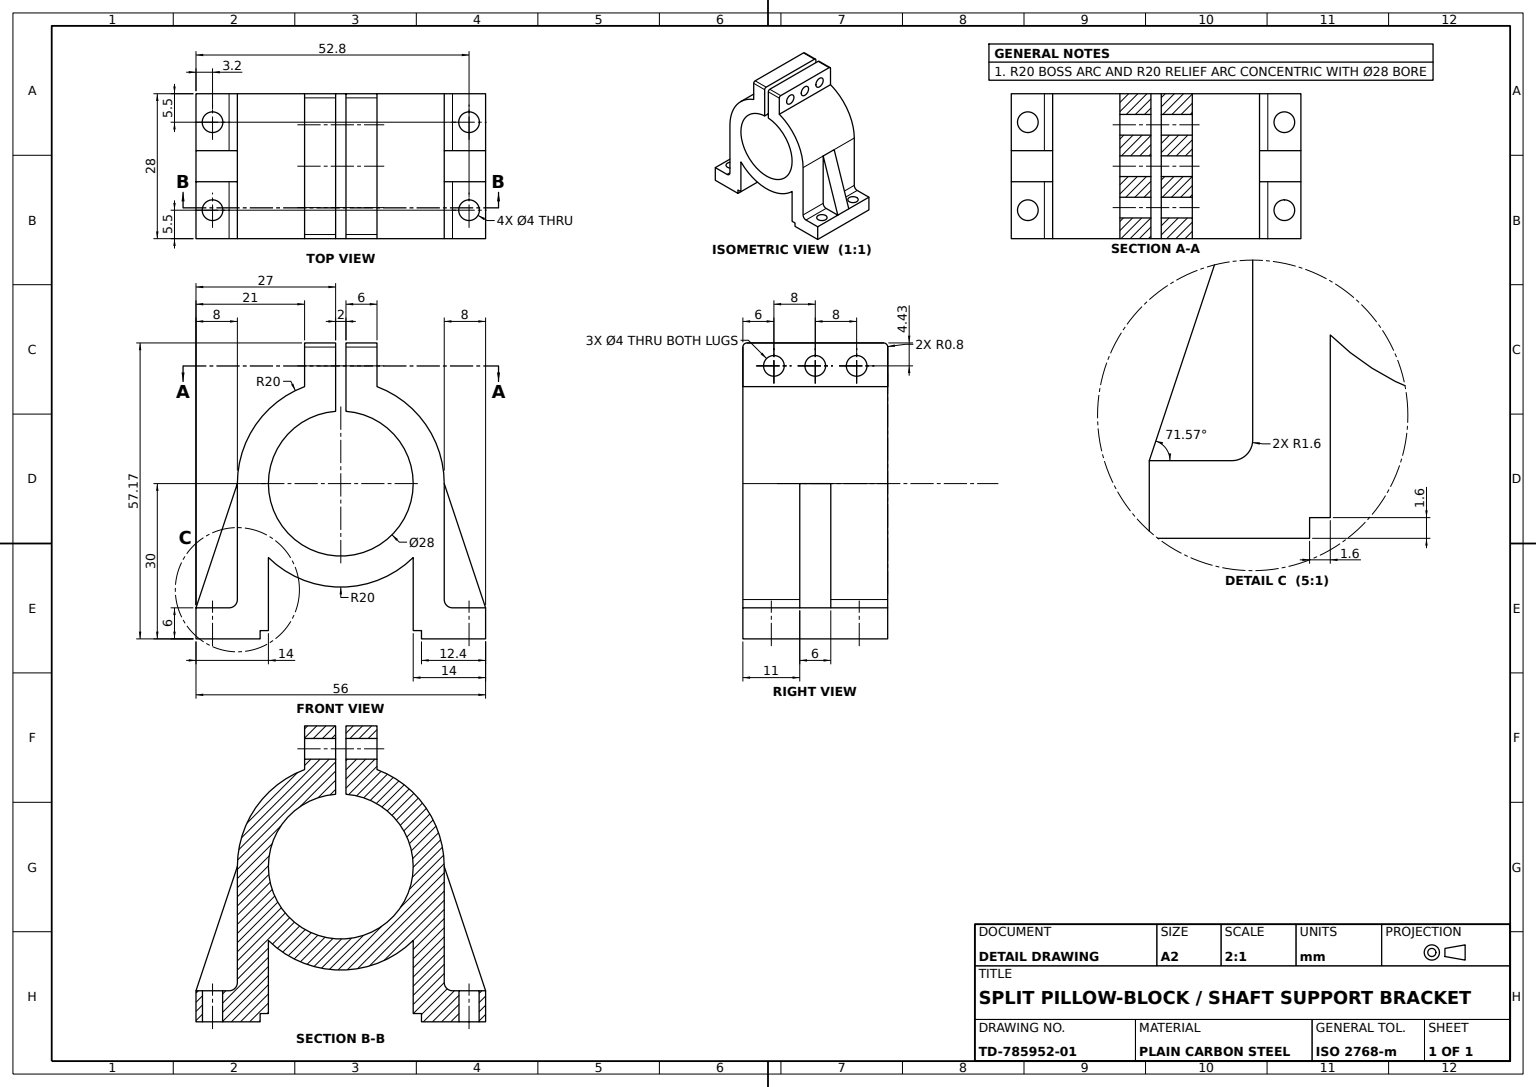
solid
v1 (-20,0,28)
v2 (-20,0,17)
e1 v1 v2 LINE
v3 (-20,-22.4,17)
e2 v3 v2 LINE
v4 (-20,-22.4,28)
e3 v3 v4 LINE
e4 v4 v1 LINE
face PLANE(AX(P(-20,0,17),D(1,0,0),D(0,0,-1))) rev [e1 -e2 e3 e4]
v5 (-28,-24,28)
v6 (-28,-24,17)
e5 v5 v6 LINE
v7 (-28,-24,11)
e6 v6 v7 LINE
v8 (-28,-24,0)
e7 v7 v8 LINE
v9 (-28,-30,0)
e8 v8 v9 LINE
v10 (-28,-30,28)
e9 v10 v9 LINE
e10 v5 v10 LINE
face PLANE(AX(P(-28,-24,28),D(1,0,0),D(0,0,-1))) rev [e5 e6 e7 e8 -e9 -e10]
v11 (-21.6,-24,11)
v12 (-21.6,-24,0)
e11 v11 v12 LINE
v13 (-20,-22.4,11)
e12 v13 v11 CIRCLE(AX(P(-21.6,-22.4,11),D(0,0,-1),D(-1,0,0)),1.6)
v14 (-20,-22.4,0)
e13 v13 v14 LINE
e14 v14 v12 CIRCLE(AX(P(-21.6,-22.4,0),D(0,0,-1),D(-1,0,0)),1.6)
face CYL(AX(P(-21.6,-22.4,11),D(0,0,-1),D(-1,0,0)),1.6) rev [-e11 -e12 e13 e14]
v15 (20,-22.4,11)
v16 (20,0,11)
e15 v15 v16 LINE
v17 (20,-22.4,0)
e16 v15 v17 LINE
v18 (20,0,0)
e17 v17 v18 LINE
e18 v16 v18 LINE
face PLANE(AX(P(20,0,11),D(-1,0,0),D(0,0,1))) rev [-e15 e16 e17 -e18]
v19 (1,27.174984,0.8)
v20 (7,27.174984,0.8)
e19 v19 v20 LINE
v21 (7,26.374984,0)
e20 v20 v21 CIRCLE(AX(P(7,26.374984,0.8),D(-1,0,0),D(0,0,-1)),0.8)
v22 (1,26.374984,0)
e21 v21 v22 LINE
e22 v19 v22 CIRCLE(AX(P(1,26.374984,0.8),D(-1,0,0),D(0,0,-1)),0.8)
face CYL(AX(P(-11,26.374984,0.8),D(1,0,0),D(0,0,-1)),0.8) [e19 e20 e21 -e22]
v23 (1,22.743733,4)
v24 (1,22.743733,8)
e23 v23 v24 CIRCLE(AX(P(1,22.743733,6),D(1,0,0),D(0,0,-1)),2)
v25 (7,22.743733,4)
e24 v23 v25 LINE
v26 (7,22.743733,8)
e25 v25 v26 CIRCLE(AX(P(7,22.743733,6),D(1,0,0),D(0,0,-1)),2)
e26 v24 v26 LINE
face CYL(AX(P(-13,22.743733,6),D(1,0,0),D(0,0,-1)),2) rev [-e23 e24 e25 -e26]
v27 (20,-22.4,17)
v28 (20,-22.4,28)
e27 v27 v28 LINE
v29 (21.6,-24,28)
e28 v28 v29 CIRCLE(AX(P(21.6,-22.4,28),D(0,0,1),D(-1,0,0)),1.6)
v30 (21.6,-24,17)
e29 v30 v29 LINE
e30 v27 v30 CIRCLE(AX(P(21.6,-22.4,17),D(0,0,1),D(-1,0,0)),1.6)
face CYL(AX(P(21.6,-22.4,17),D(0,0,1),D(1,0,0)),1.6) rev [e27 e28 -e29 -e30]
v31 (21.6,-24,11)
e31 v31 v15 CIRCLE(AX(P(21.6,-22.4,11),D(0,0,-1),D(-1,0,0)),1.6)
v32 (21.6,-24,0)
e32 v31 v32 LINE
e33 v32 v17 CIRCLE(AX(P(21.6,-22.4,0),D(0,0,-1),D(-1,0,0)),1.6)
face CYL(AX(P(21.6,-22.4,11),D(0,0,-1),D(-1,0,0)),1.6) rev [-e16 -e31 e32 e33]
v33 (24.8,-30,24.5)
v34 (24.8,-24,24.5)
e34 v33 v34 LINE
v35 (24.8,-24,20.5)
e35 v34 v35 CIRCLE(AX(P(24.8,-24,22.5),D(0,1,0),D(0,0,1)),2)
v36 (24.8,-30,20.5)
e36 v36 v35 LINE
e37 v33 v36 CIRCLE(AX(P(24.8,-30,22.5),D(0,1,0),D(0,0,1)),2)
face CYL(AX(P(24.8,-44,22.5),D(0,1,0),D(0,0,1)),2) rev [e34 e35 -e36 -e37]
v37 (28,-24,11)
e38 v16 v37 LINE
v38 (20,0,17)
e39 v38 v16 LINE
v39 (28,-24,17)
e40 v39 v38 LINE
e41 v39 v37 LINE
face PLANE(AX(P(20,0,0),D(0.948683298,0.316227766,0),D(-0.316227766,0.948683298,0))) [-e38 -e39 -e40 e41]
v40 (24.8,-30,3.5)
v41 (24.8,-30,7.5)
e42 v40 v41 CIRCLE(AX(P(24.8,-30,5.5),D(0,1,0),D(0,0,1)),2)
v42 (24.8,-24,3.5)
e43 v40 v42 LINE
v43 (24.8,-24,7.5)
e44 v42 v43 CIRCLE(AX(P(24.8,-24,5.5),D(0,1,0),D(0,0,1)),2)
e45 v41 v43 LINE
face CYL(AX(P(24.8,-44,5.5),D(0,1,0),D(0,0,1)),2) rev [-e42 e43 e44 -e45]
v44 (-14,-14.282857,0)
v45 (14,-14.282857,0)
e46 v44 v45 CIRCLE(AX(P(0,0,0),D(0,0,1),D(1,0,0)),20)
v46 (14,-14.282857,28)
e47 v46 v45 LINE
v47 (-14,-14.282857,28)
e48 v47 v46 CIRCLE(AX(P(0,0,28),D(0,0,1),D(1,0,0)),20)
e49 v47 v44 LINE
face CYL(AX(P(0,0,28),D(0,0,-1),D(-1,0,0)),20) [e46 -e47 -e48 e49]
v48 (-21.6,-24,17)
v49 (-21.6,-24,28)
e50 v48 v49 LINE
e51 v49 v4 CIRCLE(AX(P(-21.6,-22.4,28),D(0,0,1),D(-1,0,0)),1.6)
e52 v48 v3 CIRCLE(AX(P(-21.6,-22.4,17),D(0,0,1),D(-1,0,0)),1.6)
face CYL(AX(P(-21.6,-22.4,17),D(0,0,1),D(1,0,0)),1.6) rev [e50 e51 -e3 -e52]
v50 (-7,26.374984,28)
v51 (-7,27.174984,27.2)
e53 v50 v51 CIRCLE(AX(P(-7,26.374984,27.2),D(-1,0,0),D(0,0,-1)),0.8)
v52 (-1,26.374984,28)
e54 v52 v50 LINE
v53 (-1,27.174984,27.2)
e55 v53 v52 CIRCLE(AX(P(-1,26.374984,27.2),D(1,0,0),D(0,0,1)),0.8)
e56 v51 v53 LINE
face CYL(AX(P(-11,26.374984,27.2),D(1,0,0),D(0,0,-1)),0.8) [-e53 -e54 -e55 -e56]
e57 v35 v34 CIRCLE(AX(P(24.8,-24,22.5),D(0,1,0),D(0,0,1)),2)
v54 (28,-24,28)
e58 v29 v54 LINE
e59 v54 v39 LINE
e60 v30 v39 LINE
face PLANE(AX(P(28,-24,17),D(0,-1,0),D(0,0,-1))) rev [-e35 -e57] [e58 e59 -e60 e29]
e61 v43 v42 CIRCLE(AX(P(24.8,-24,5.5),D(0,1,0),D(0,0,1)),2)
e62 v41 v40 CIRCLE(AX(P(24.8,-30,5.5),D(0,1,0),D(0,0,1)),2)
face CYL(AX(P(24.8,-44,5.5),D(0,1,0),D(0,0,1)),2) rev [e45 e61 -e43 -e62]
v55 (1,22.743733,16)
v56 (7,22.743733,16)
e63 v55 v56 LINE
v57 (7,22.743733,12)
e64 v56 v57 CIRCLE(AX(P(7,22.743733,14),D(1,0,0),D(0,0,-1)),2)
v58 (1,22.743733,12)
e65 v58 v57 LINE
e66 v55 v58 CIRCLE(AX(P(1,22.743733,14),D(1,0,0),D(0,0,-1)),2)
face CYL(AX(P(-13,22.743733,14),D(1,0,0),D(0,0,-1)),2) rev [e63 e64 -e65 -e66]
e67 v57 v56 CIRCLE(AX(P(7,22.743733,14),D(1,0,0),D(0,0,-1)),2)
e68 v58 v55 CIRCLE(AX(P(1,22.743733,14),D(1,0,0),D(0,0,-1)),2)
face CYL(AX(P(-13,22.743733,14),D(1,0,0),D(0,0,-1)),2) rev [e67 -e63 -e68 e65]
v59 (-15.6,-30,28)
v60 (-15.6,-30,0)
e69 v59 v60 LINE
v61 (-15.6,-28.4,0)
e70 v60 v61 LINE
v62 (-15.6,-28.4,28)
e71 v62 v61 LINE
e72 v59 v62 LINE
face PLANE(AX(P(-15.6,-30,28),D(-1,0,0),D(0,0,1))) rev [e69 e70 -e71 -e72]
v63 (1,13.96424,28)
v64 (1,13.96424,0)
e73 v63 v64 LINE
v65 (14,0,0)
e74 v64 v65 CIRCLE(AX(P(0,0,0),D(0,0,-1),D(1,0,0)),14)
v66 (14,0,28)
e75 v66 v65 LINE
e76 v63 v66 CIRCLE(AX(P(0,0,28),D(0,0,-1),D(1,0,0)),14)
face CYL(AX(P(0,0,28),D(0,0,-1),D(-1,0,0)),14) rev [e73 e74 -e75 -e76]
v67 (-7,22.743733,20)
v68 (-1,22.743733,20)
e77 v67 v68 LINE
v69 (-1,22.743733,24)
e78 v69 v68 CIRCLE(AX(P(-1,22.743733,22),D(-1,0,0),D(0,0,1)),2)
v70 (-7,22.743733,24)
e79 v70 v69 LINE
e80 v67 v70 CIRCLE(AX(P(-7,22.743733,22),D(1,0,0),D(0,0,-1)),2)
face CYL(AX(P(-13,22.743733,22),D(1,0,0),D(0,0,-1)),2) rev [e77 -e78 -e79 -e80]
v71 (7,22.743733,20)
v72 (7,22.743733,24)
e81 v71 v72 CIRCLE(AX(P(7,22.743733,22),D(1,0,0),D(0,0,-1)),2)
v73 (1,22.743733,24)
e82 v73 v72 LINE
v74 (1,22.743733,20)
e83 v74 v73 CIRCLE(AX(P(1,22.743733,22),D(1,0,0),D(0,0,-1)),2)
e84 v74 v71 LINE
face CYL(AX(P(-13,22.743733,22),D(1,0,0),D(0,0,-1)),2) rev [e81 -e82 -e83 e84]
v75 (-20,0,11)
e85 v2 v75 LINE
e86 v7 v75 LINE
e87 v2 v6 LINE
face PLANE(AX(P(-20,0,28),D(-0.948683298,0.316227766,0),D(-0.316227766,-0.948683298,0))) [e85 -e86 -e6 -e87]
e88 v68 v69 CIRCLE(AX(P(-1,22.743733,22),D(-1,0,0),D(0,0,1)),2)
e89 v70 v67 CIRCLE(AX(P(-7,22.743733,22),D(1,0,0),D(0,0,-1)),2)
face CYL(AX(P(-13,22.743733,22),D(1,0,0),D(0,0,-1)),2) rev [e79 -e88 -e77 -e89]
v76 (1,26.374984,28)
e90 v76 v63 LINE
v77 (-14,0,28)
e91 v66 v77 CIRCLE(AX(P(0,0,28),D(0,0,-1),D(1,0,0)),14)
v78 (-1,13.96424,28)
e92 v77 v78 CIRCLE(AX(P(0,0,28),D(0,0,-1),D(1,0,0)),14)
e93 v78 v52 LINE
v79 (-7,18.734994,28)
e94 v50 v79 LINE
e95 v79 v1 CIRCLE(AX(P(0,0,28),D(0,0,1),D(1,0,0)),20)
e96 v5 v49 LINE
e97 v10 v59 LINE
v80 (-14,-28.4,28)
e98 v62 v80 LINE
e99 v80 v47 LINE
v81 (14,-28.4,28)
e100 v46 v81 LINE
v82 (15.6,-28.4,28)
e101 v81 v82 LINE
v83 (15.6,-30,28)
e102 v82 v83 LINE
v84 (28,-30,28)
e103 v83 v84 LINE
e104 v84 v54 LINE
v85 (20,0,28)
e105 v85 v28 LINE
v86 (7,18.734994,28)
e106 v85 v86 CIRCLE(AX(P(0,0,28),D(0,0,1),D(1,0,0)),20)
v87 (7,26.374984,28)
e107 v86 v87 LINE
e108 v87 v76 LINE
face PLANE(AX(P(0,0,28),D(0,0,1),D(1,0,0))) [e90 e76 e91 e92 e93 e54 e94 e95 -e4 -e51 -e96 e10 e97 e72 e98 e99 e48 e100 e101 e102 e103 e104 -e58 -e28 -e105 e106 e107 e108]
v88 (-24.8,-24,20.5)
v89 (-24.8,-24,24.5)
e109 v88 v89 CIRCLE(AX(P(-24.8,-24,22.5),D(0,1,0),D(0,0,1)),2)
e110 v89 v88 CIRCLE(AX(P(-24.8,-24,22.5),D(0,1,0),D(0,0,1)),2)
e111 v6 v48 LINE
face PLANE(AX(P(-21.6,-24,17),D(0,-1,0),D(0,0,-1))) rev [-e109 -e110] [-e50 -e111 -e5 e96]
v90 (28,-30,0)
v91 (28,-24,0)
e112 v90 v91 LINE
e113 v37 v91 LINE
e114 v84 v90 LINE
face PLANE(AX(P(28,-24,28),D(-1,0,0),D(0,0,1))) rev [e112 -e113 -e41 -e59 -e104 e114]
e115 v36 v33 CIRCLE(AX(P(24.8,-30,22.5),D(0,1,0),D(0,0,1)),2)
face CYL(AX(P(24.8,-44,22.5),D(0,1,0),D(0,0,1)),2) rev [e57 -e34 -e115 e36]
v92 (-1,26.374984,0)
v93 (-1,27.174984,0.8)
e116 v92 v93 CIRCLE(AX(P(-1,26.374984,0.8),D(1,0,0),D(0,0,1)),0.8)
v94 (-7,26.374984,0)
e117 v92 v94 LINE
v95 (-7,27.174984,0.8)
e118 v95 v94 CIRCLE(AX(P(-7,26.374984,0.8),D(-1,0,0),D(0,0,-1)),0.8)
e119 v95 v93 LINE
face CYL(AX(P(-11,26.374984,0.8),D(1,0,0),D(0,0,-1)),0.8) [-e116 e117 -e118 e119]
v96 (-14,-28.4,0)
e120 v61 v96 LINE
e121 v80 v96 LINE
face PLANE(AX(P(-15.6,-28.4,28),D(0,1,0),D(0,0,1))) rev [e71 e120 -e121 -e98]
v97 (14,-28.4,0)
e122 v45 v97 LINE
e123 v81 v97 LINE
face PLANE(AX(P(14,-28.4,28),D(1,0,0),D(0,0,-1))) rev [e122 -e123 -e100 e47]
v98 (15.6,-28.4,0)
e124 v97 v98 LINE
e125 v82 v98 LINE
face PLANE(AX(P(15.6,-28.4,28),D(0,1,0),D(0,0,1))) rev [e124 -e125 -e101 e123]
v99 (-1,22.743733,16)
v100 (-1,22.743733,12)
e126 v99 v100 CIRCLE(AX(P(-1,22.743733,14),D(-1,0,0),D(0,0,1)),2)
v101 (-7,22.743733,16)
e127 v101 v99 LINE
v102 (-7,22.743733,12)
e128 v102 v101 CIRCLE(AX(P(-7,22.743733,14),D(1,0,0),D(0,0,-1)),2)
e129 v102 v100 LINE
face CYL(AX(P(-13,22.743733,14),D(1,0,0),D(0,0,-1)),2) rev [-e126 -e127 -e128 e129]
face PLANE(AX(P(-21.6,-22.4,17),D(0,0,-1),D(-1,0,0))) rev [e87 e111 e52 e2]
e130 v85 v38 LINE
e131 v38 v27 LINE
face PLANE(AX(P(20,-22.4,17),D(-1,0,0),D(0,0,1))) rev [-e130 e105 -e27 -e131]
v103 (-7,18.734994,0)
e132 v79 v103 LINE
v104 (-20,0,0)
e133 v103 v104 CIRCLE(AX(P(0,0,0),D(0,0,1),D(1,0,0)),20)
e134 v75 v104 LINE
face CYL(AX(P(0,0,28),D(0,0,-1),D(-1,0,0)),20) [e132 e133 -e134 -e85 -e1 -e95]
e135 v73 v74 CIRCLE(AX(P(1,22.743733,22),D(1,0,0),D(0,0,-1)),2)
e136 v24 v23 CIRCLE(AX(P(1,22.743733,6),D(1,0,0),D(0,0,-1)),2)
v105 (1,27.174984,27.2)
e137 v105 v19 LINE
e138 v22 v64 LINE
e139 v76 v105 CIRCLE(AX(P(1,26.374984,27.2),D(-1,0,0),D(0,0,-1)),0.8)
face PLANE(AX(P(1,19.974984,28),D(1,0,0),D(0,0,-1))) rev [e135 e83] [e66 e68] [e136 e23] [e137 e22 e138 -e73 -e90 e139]
e140 v37 v31 LINE
face PLANE(AX(P(21.6,-22.4,11),D(0,0,-1),D(-1,0,0))) [e38 e140 e31 e15]
v106 (7,27.174984,27.2)
e141 v106 v20 LINE
e142 v87 v106 CIRCLE(AX(P(7,26.374984,27.2),D(-1,0,0),D(0,0,-1)),0.8)
v107 (7,18.734994,0)
e143 v86 v107 LINE
e144 v107 v21 LINE
e145 v72 v71 CIRCLE(AX(P(7,22.743733,22),D(1,0,0),D(0,0,-1)),2)
e146 v26 v25 CIRCLE(AX(P(7,22.743733,6),D(1,0,0),D(0,0,-1)),2)
face PLANE(AX(P(7,27.174984,28),D(-1,0,0),D(0,0,1))) rev [-e67 -e64] [-e20 -e141 -e142 -e107 e143 e144] [-e145 -e81] [-e146 -e25]
e147 v18 v107 CIRCLE(AX(P(0,0,0),D(0,0,1),D(1,0,0)),20)
face CYL(AX(P(0,0,28),D(0,0,-1),D(-1,0,0)),20) [e147 -e143 -e106 e130 e39 e18]
e148 v105 v106 LINE
face CYL(AX(P(-11,26.374984,27.2),D(1,0,0),D(0,0,-1)),0.8) [-e108 e142 -e148 -e139]
e149 v91 v32 LINE
v108 (15.6,-30,0)
e150 v108 v90 LINE
e151 v98 v108 LINE
e152 v96 v44 LINE
e153 v9 v60 LINE
e154 v12 v8 LINE
e155 v104 v14 LINE
e156 v94 v103 LINE
v109 (-1,13.96424,0)
e157 v109 v92 LINE
v110 (-14,0,0)
e158 v110 v109 CIRCLE(AX(P(0,0,0),D(0,0,-1),D(1,0,0)),14)
e159 v65 v110 CIRCLE(AX(P(0,0,0),D(0,0,-1),D(1,0,0)),14)
face PLANE(AX(P(0,0,0),D(0,0,1),D(1,0,0))) rev [-e74 -e138 -e21 -e144 -e147 -e17 -e33 -e149 -e112 -e150 -e151 -e124 -e122 -e46 -e152 -e120 -e70 -e153 -e8 -e154 -e14 -e155 -e133 -e156 -e117 -e157 -e158 -e159]
face CYL(AX(P(-13,22.743733,6),D(1,0,0),D(0,0,-1)),2) rev [e146 -e24 -e136 e26]
v111 (-24.8,-30,7.5)
v112 (-24.8,-24,7.5)
e160 v111 v112 LINE
v113 (-24.8,-30,3.5)
e161 v113 v111 CIRCLE(AX(P(-24.8,-30,5.5),D(0,1,0),D(0,0,1)),2)
v114 (-24.8,-24,3.5)
e162 v113 v114 LINE
e163 v114 v112 CIRCLE(AX(P(-24.8,-24,5.5),D(0,1,0),D(0,0,1)),2)
face CYL(AX(P(-24.8,-44,5.5),D(0,1,0),D(0,0,1)),2) rev [-e160 -e161 e162 e163]
v115 (-7,22.743733,4)
v116 (-1,22.743733,4)
e164 v115 v116 LINE
v117 (-7,22.743733,8)
e165 v117 v115 CIRCLE(AX(P(-7,22.743733,6),D(1,0,0),D(0,0,-1)),2)
v118 (-1,22.743733,8)
e166 v117 v118 LINE
e167 v116 v118 CIRCLE(AX(P(-1,22.743733,6),D(-1,0,0),D(0,0,1)),2)
face CYL(AX(P(-13,22.743733,6),D(1,0,0),D(0,0,-1)),2) rev [-e164 -e165 e166 -e167]
face PLANE(AX(P(1,27.174984,28),D(0,-1,0),D(0,0,-1))) rev [e141 -e19 -e137 e148]
e168 v101 v102 CIRCLE(AX(P(-7,22.743733,14),D(1,0,0),D(0,0,-1)),2)
e169 v100 v99 CIRCLE(AX(P(-1,22.743733,14),D(-1,0,0),D(0,0,1)),2)
face CYL(AX(P(-13,22.743733,14),D(1,0,0),D(0,0,-1)),2) rev [-e129 -e168 e127 -e169]
e170 v75 v13 LINE
face PLANE(AX(P(-20,0,11),D(1,0,0),D(0,0,-1))) rev [e155 -e13 -e170 e134]
e171 v53 v93 LINE
e172 v51 v95 LINE
face PLANE(AX(P(-1,27.174984,28),D(0,-1,0),D(0,0,-1))) rev [e171 -e119 -e172 e56]
e173 v115 v117 CIRCLE(AX(P(-7,22.743733,6),D(1,0,0),D(0,0,-1)),2)
face PLANE(AX(P(-7,27.174984,28),D(1,0,0),D(0,0,-1))) rev [e165 e173] [e156 -e132 -e94 e53 e172 e118] [e168 e128] [e89 e80]
e174 v77 v110 LINE
face CYL(AX(P(0,0,28),D(0,0,-1),D(-1,0,0)),14) rev [e159 -e174 -e91 e75]
face CYL(AX(P(-13,22.743733,22),D(1,0,0),D(0,0,-1)),2) rev [-e84 -e135 e82 e145]
e175 v111 v113 CIRCLE(AX(P(-24.8,-30,5.5),D(0,1,0),D(0,0,1)),2)
v119 (-24.8,-30,20.5)
v120 (-24.8,-30,24.5)
e176 v119 v120 CIRCLE(AX(P(-24.8,-30,22.5),D(0,1,0),D(0,0,1)),2)
e177 v120 v119 CIRCLE(AX(P(-24.8,-30,22.5),D(0,1,0),D(0,0,1)),2)
face PLANE(AX(P(-28,-30,28),D(0,1,0),D(0,0,1))) rev [e153 -e69 -e97 e9] [e175 e161] [e176 e177]
face PLANE(AX(P(21.6,-24,11),D(0,-1,0),D(0,0,-1))) rev [-e44 -e61] [-e32 -e140 e113 e149]
e178 v11 v7 LINE
e179 v112 v114 CIRCLE(AX(P(-24.8,-24,5.5),D(0,1,0),D(0,0,1)),2)
face PLANE(AX(P(-21.6,-24,11),D(0,-1,0),D(0,0,-1))) rev [e11 e154 -e7 -e178] [-e179 -e163]
e180 v118 v116 CIRCLE(AX(P(-1,22.743733,6),D(-1,0,0),D(0,0,1)),2)
face CYL(AX(P(-13,22.743733,6),D(1,0,0),D(0,0,-1)),2) rev [-e166 -e173 e164 -e180]
e181 v83 v108 LINE
face PLANE(AX(P(15.6,-30,28),D(1,0,0),D(0,0,-1))) rev [-e102 e125 e151 -e181]
e182 v120 v89 LINE
e183 v119 v88 LINE
face CYL(AX(P(-24.8,-44,22.5),D(0,1,0),D(0,0,1)),2) rev [-e177 e182 e110 -e183]
face PLANE(AX(P(28,-30,28),D(0,1,0),D(0,0,1))) rev [-e114 -e103 e181 e150] [e37 e115] [e62 e42]
e184 v78 v109 LINE
face PLANE(AX(P(-1,19.974984,28),D(-1,0,0),D(0,0,1))) rev [e167 e180] [e116 -e171 e55 -e93 e184 e157] [e88 e78] [e169 e126]
face PLANE(AX(P(21.6,-22.4,17),D(0,0,-1),D(-1,0,0))) rev [e40 e131 e30 e60]
face PLANE(AX(P(-14,-28.4,28),D(-1,0,0),D(0,0,1))) rev [-e49 -e99 e121 e152]
face CYL(AX(P(-24.8,-44,22.5),D(0,1,0),D(0,0,1)),2) rev [-e176 e183 e109 -e182]
face CYL(AX(P(0,0,28),D(0,0,-1),D(-1,0,0)),14) rev [-e92 e174 e158 -e184]
face PLANE(AX(P(-21.6,-22.4,11),D(0,0,-1),D(-1,0,0))) [e178 e86 e170 e12]
face CYL(AX(P(-24.8,-44,5.5),D(0,1,0),D(0,0,1)),2) rev [e160 e179 -e162 -e175]
